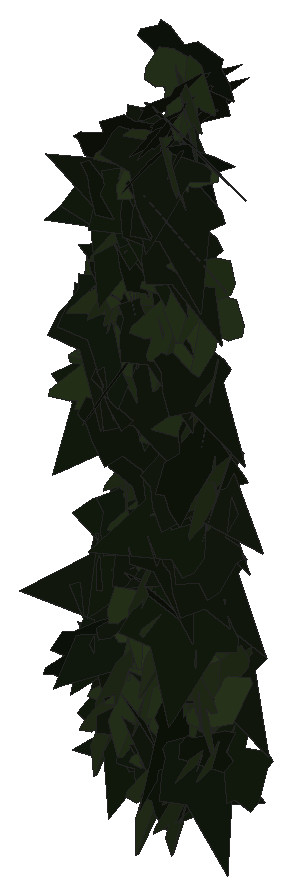
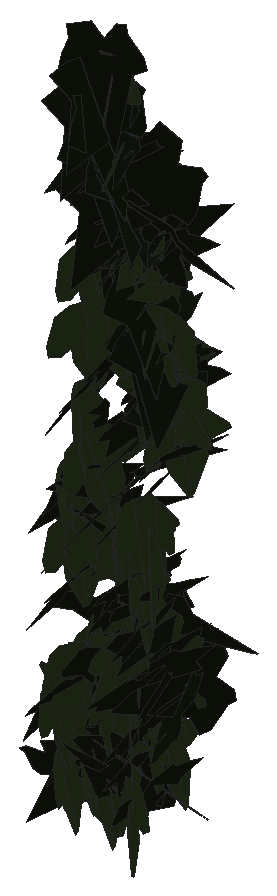
# SketchUp Ruby script. Lengths in inches.
U = 1.inch
M = Sketchup.active_model
def pt(a) = Geom::Point3d.new(a.map { |v| v * U })
def face(e, loops, mat)
  f = e.add_face(loops[0].map { |a| pt(a) })
  loops[1..].each { |l| e.add_face(l.map { |a| pt(a) }).erase! }
  f.material = f.back_material = mat if mat
  f
end
# faces: each face lists its corners as indices into pts; further lists are holes
def faces(e, pts, list, mat = nil) = list.each { |f| face(e, (f[0].is_a?(Array) ? f : [f]).map { |l| l.map { |i| pts[i] } }, mat) }
# xy, xz, yz: faces in a plane at the given z, y or x. An outline is a flat list of corners, or four numbers for a rectangle; further outlines are holes
def ring(l) = l.size == 4 ? [[l[0], l[1]], [l[2], l[1]], [l[2], l[3]], [l[0], l[3]]] : l.each_slice(2).to_a
def flat(e, list, mat, &to3) = list.each { |f| face(e, (f[0].is_a?(Array) ? f : [f]).map { |l| ring(l).map { |u, v| to3.(u, v) } }, mat) }
def xy(e, z, list, mat = nil) = flat(e, list, mat) { |x, y| [x, y, z] }
def xz(e, y, list, mat = nil) = flat(e, list, mat) { |x, z| [x, y, z] }
def yz(e, x, list, mat = nil) = flat(e, list, mat) { |y, z| [x, y, z] }
def lines(e, pts, list) = list.each { |a, b| e.add_line(pt(pts[a]), pt(pts[b])) }
# prism: a flat outline (further loops are holes) pulled along v
def prism(e, loops, v, mat = nil)
  f = face(e, loops, mat); d = Geom::Vector3d.new(v.map { |x| x * U })
  f.pushpull(f.normal.samedirection?(d) ? d.length : -d.length)
end
def box(e, o, s, mat = nil) = prism(e, [[o, [o[0] + s[0], o[1], o[2]], [o[0] + s[0], o[1] + s[1], o[2]], [o[0], o[1] + s[1], o[2]]]], [0, 0, s[2]], mat)
def at(x, y, z, deg = 0) = Geom::Transformation.translation(pt([x, y, z])) * Geom::Transformation.rotation(ORIGIN, Z_AXIS, deg.degrees)
def axes(o, x, y, z) = Geom::Transformation.new([*x, 0, *y, 0, *z, 0, *pt(o).to_a, 1])
def part(name) = M.definitions.add(name)
# library, detail: a bought-in or finely detailed component or shape, given as its bounding box
def library(name, o, s) = part(name).tap { |d| box(d.entities, o, s) }
def detail(e, o, s) = box(e.add_group.entities, o, s)
def put(e, d, t, mat = nil) = e.add_instance(d, t).tap { |i| i.material = mat if mat }
def group(e, t, mat = nil) = e.add_group.tap { |g| g.transformation = t; g.material = mat if mat }.entities
root = M.entities
M.materials.add("efeu1").color = [18, 25, 13]
M.materials.add("efeu2").color = [43, 57, 29]
c1 = part("ivyleaf_9")
p = [[1.54,2.16,1.25],[1.36,2.04,1.19],[-0.21,0.99,0.68],[-0.71,1.11,0.82],[-0.85,0.86,0.67],[-0.8,0.17,0.21],
  [-0.9,-0.01,0.1],[-0.67,-0.16,-0.02],[-0.08,-0.08,-0.05],[-0.03,-0.6,-0.4],[0.65,-0.88,-0.66],[0.83,-0.6,-0.49],
  [1.29,-0.42,-0.43],[1.8125,-0.07,-0.26],[1.21,0.44,0.15]]
faces(c1.entities,p,[[0,1,2,3,4,5,6,7,8,9,10,11,12,13,14]],"efeu1")
c2 = part("ivyleaf_10")
p = [[0,0.5,-0.03],[-0.0625,2.02,-0.43],[-0.19,2.01,-0.46],[-0.54,1.05,-0.29],[-0.52,0.625,-0.18],[-0.83,0.76,-0.28],
  [-1.16,0.64,-0.33],[-1.15,0.33,-0.24],[-0.77,-0.39,0.02],[-0.3,-0.51,0.16],[0.04,-0.48,0.23],[-0.02,2.01,-0.4375],
  [-0.06,2.01,-0.43],[0.04,-0.49,0.23],[0.67,-0.49,0.14],[1.38,0.36,-0.2],[1.375,0.51,-0.24],[0.81,0.65,-0.19],
  [0.62,0.59,-0.15],[0.6,1.09,-0.28],[0.5,1.23,-0.31]]
faces(c2.entities,p,[[0,1,2,3,4,5,6,7,8,9,10],[11,12,0,13,14,15,16,17,18,19,20]],"efeu2")
put(root,c1,axes([14.96,224.05,229.89],[0.063,0.49565,0.01912],[-0.02815,0.02282,-0.49869],[-0.49522,0.06176,0.03078]))
put(root,c1,axes([15.22,223.91,225.72],[-0.39113,0.07566,0.30215],[-0.30173,0.02832,-0.39769],[-0.07729,-0.49343,0.0235]))
put(root,c2,axes([14.84,224.45,226.98],[0.34673,-0.34178,-0.11385],[0.0087,0.16592,-0.47159],[0.36014,0.32505,0.12101]))
put(root,c2,axes([15.23,223.79,228.77],[-0.07541,0.02724,0.49353],[-0.4942,-0.01303,-0.0748],[0.00879,-0.49909,0.02889]))
put(root,c2,axes([14.91,223.86,228.55],[-0.22304,-0.43361,0.11063],[0.0193,-0.13282,-0.48165],[0.44708,-0.21058,0.07599]))
put(root,c1,axes([14.65,223.47,224.73],[0.28736,0.2041,0.35464],[0.2644,0.23812,-0.35128],[-0.31228,0.38942,0.02893]))
put(root,c1,axes([14.9,224.4,225.13],[-0.24918,-0.40137,0.16373],[-0.04775,-0.16229,-0.47051],[0.43085,-0.25012,0.04255]))
put(root,c2,axes([14.92,224.08,223.89],[0.07183,-0.47806,0.12768],[0.03312,-0.12408,-0.48323],[0.4937,0.07788,0.01384]))
put(root,c2,axes([14.95,224.15,227.26],[0.34077,-0.30537,-0.20156],[-0.04793,0.23581,-0.43829],[0.36274,0.31803,0.13144]))
put(root,c1,axes([14.82,224.625,223.45],[-0.09691,-0.47403,0.12613],[-0.01843,-0.12496,-0.48378],[0.49017,-0.09841,0.00674]))
put(root,c1,axes([14.93,224.125,228.18],[-0.28894,-0.35601,0.19943],[-0.00668,-0.2402,-0.43847],[0.408,-0.25605,0.13405]))
put(root,c2,axes([14.75,224.14,229.35],[0.32621,0.31913,0.2043],[0.11757,0.17103,-0.45489],[-0.36022,0.34482,0.03654]))
put(root,c2,axes([14.93,224.78,223.4],[0.37932,-0.2878,-0.1526],[-0.0287,0.20379,-0.45568],[0.32449,0.35446,0.13808]))
put(root,c2,axes([14.99,224.04,229.71],[-0.15997,-0.46885,0.06775],[0.00767,-0.07406,-0.49442],[0.47366,-0.15715,0.03088]))
put(root,c1,axes([14.625,224.17,224.48],[0.31864,-0.36062,0.13572],[0.08272,-0.10799,-0.48114],[0.37633,0.32907,-0.00916]))
put(root,c1,axes([14.86,224.1,229.35],[-0.1462,-0.47355,-0.06618],[0.00774,0.06685,-0.49545],[0.47809,-0.14589,-0.01222]))
put(root,c2,axes([15.01,224.49,226.56],[0.11234,-0.48242,-0.06822],[0.0009,0.07022,-0.49504],[0.48722,0.1111,0.01665]))
put(root,c2,axes([14.98,223.97,229.91],[0.36157,-0.34351,-0.03562],[-0.02197,0.02859,-0.4987],[0.34465,0.3622,0.00558]))
put(root,c1,axes([15.11,224,229.86],[0.03322,0.48974,0.09515],[-0.013,0.09618,-0.49049],[-0.49873,0.03011,0.01912]))
put(root,c1,axes([14.98,224.51,226.22],[-0.25217,-0.40835,0.1402],[0.00224,-0.1636,-0.47247],[0.43174,-0.23766,0.08434]))
put(root,c2,axes([14.91,224.1,230.11],[-0.45836,-0.03724,-0.19626],[0.19586,0.01291,-0.45986],[0.03932,-0.49844,0.00275]))
put(root,c1,axes([15.06,224.125,225.07],[-0.22004,-0.33771,0.29586],[-0.11073,-0.27849,-0.40023],[0.43511,-0.24166,0.04777]))
put(root,c2,axes([15.07,224.04,229.9375],[0.05078,-0.49639,-0.03196],[-0.00004,0.03212,-0.49897],[0.49741,0.05068,0.00322]))
put(root,c2,axes([15.2,224.04,224.49],[-0.39676,-0.25674,0.1633],[-0.12856,-0.10177,-0.47235],[0.27578,-0.41681,0.01474]))
put(root,c1,axes([14.93,224.03,224.83],[0.2535,-0.32237,-0.28603],[-0.19108,0.21337,-0.40983],[0.3863,0.31709,-0.01502]))
put(root,c1,axes([14.92,224.09,229.53],[-0.05922,-0.4947,-0.042],[-0.0005,0.04235,-0.4982],[0.49648,-0.05896,-0.00551]))
put(root,c2,axes([15.03,224.11,229.85],[0.38856,-0.30945,-0.05711],[0.00482,0.09658,-0.49056],[0.31464,0.38067,0.07804]))
put(root,c2,axes([15.13,224.41,227.34],[-0.02667,-0.49752,-0.04199],[-0.01602,0.04288,-0.4979],[0.49903,-0.02521,-0.01822]))
put(root,c2,axes([15.13,224.02,230.03],[-0.28656,0.40933,0.01831],[-0.0453,-0.00944,-0.49785],[-0.40722,-0.28699,0.0425]))
put(root,c1,axes([14.91,224.4,225.87],[0.14941,-0.47135,-0.0742],[-0.01358,0.07352,-0.49438],[0.47696,0.14974,0.00917]))
put(root,c2,axes([15.17,224,225.18],[0.34578,0.35267,0.07784],[-0.05693,-0.0532,0.49389],[0.35664,-0.35042,0.00336]))
put(root,c1,axes([15.48,223.85,231.43],[-0.45026,0.12068,0.18083],[-0.17917,0.02955,-0.46586],[-0.12312,-0.48432,0.01663]))
put(root,c1,axes([15.32,223.98,230.52],[-0.07005,0.49485,0.01483],[-0.00112,0.01482,-0.49978],[-0.49507,-0.07005,-0.00097]))
put(root,c1,axes([14.96,224.4,223.91],[0.12104,-0.47489,-0.09916],[-0.00343,0.10136,-0.48961],[0.48512,0.1192,0.02128]))
put(root,c2,axes([15.22,224.37,224.14],[0.18163,-0.42331,-0.19447],[-0.02706,0.19879,-0.45799],[0.46506,0.1769,0.0493]))
put(root,c1,axes([14.86,224,230.07],[0.31194,-0.38416,0.07154],[0.08818,-0.01997,-0.49176],[0.38068,0.31941,0.05529]))
put(root,c1,axes([15.01,224.37,224.29],[0.05807,-0.49533,-0.03577],[-0.00035,0.03597,-0.4987],[0.49662,0.05794,0.00383]))
put(root,c1,axes([15.5625,224.29,223.56],[-0.40912,0.21874,0.18648],[-0.21023,-0.00648,-0.45361],[-0.19603,-0.44957,0.09727]))
put(root,c1,axes([15.52,223.99,231.15],[-0.04477,-0.00173,0.49799],[-0.49581,-0.04663,-0.04474],[0.0466,-0.49782,0.00246]))
put(root,c1,axes([15.23,223.39,228.59],[0.16105,0.15924,0.44576],[0.07656,0.45589,-0.19052],[-0.46712,0.12962,0.12246]))
put(root,c1,axes([15,224.58,225.02],[0.15008,-0.43164,-0.2029],[0.05278,0.22643,-0.44266],[0.47402,0.11145,0.11353]))
put(root,c1,axes([15.23,224,231.19],[-0.2588,-0.42569,-0.04263],[0.01166,0.04278,-0.49803],[0.42765,-0.25877,-0.01221]))
put(root,c2,axes([15.3,223.84,224.73],[0.05533,-0.48125,-0.12383],[0.00234,0.12485,-0.48416],[0.49692,0.05299,0.01607]))
put(root,c1,axes([15.03,224.4,226.55],[0.13227,-0.45362,-0.16352],[0.05024,0.1816,-0.46314],[0.47956,0.10608,0.09362]))
put(root,c1,axes([15.04,223.73,228.23],[0.33176,-0.32221,-0.19004],[-0.04944,0.21401,-0.44917],[0.37079,0.31683,0.11014]))
put(root,c1,axes([15.02,223.86,231.39],[0.27702,-0.41617,-0.00811],[0.02374,0.02552,-0.49878],[0.41557,0.27596,0.0339]))
put(root,c1,axes([15.08,223.9375,228.7],[0.34175,-0.29492,-0.215],[-0.06128,0.244,-0.4321],[0.35979,0.32169,0.13063]))
put(root,c2,axes([15.42,224.03,224.29],[-0.23049,-0.40968,0.17039],[-0.04048,-0.17179,-0.46781],[0.44185,-0.22945,0.04603]))
put(root,c2,axes([15.25,223.87,230.37],[0.06203,0.46464,0.17395],[0.00299,0.17496,-0.46838],[-0.49613,0.05915,0.01892]))
put(root,c2,axes([15.38,223.95,230.77],[-0.12653,-0.48363,-0.00932],[0.00861,0.00739,-0.49987],[0.48365,-0.12666,0.00646]))
put(root,c2,axes([15.68,223.76,229.91],[-0.19398,0.08933,0.45209],[-0.44008,0.10966,-0.2105],[-0.13676,-0.47958,0.03608]))
put(root,c2,axes([15.41,223.74,231.4375],[-0.42031,0.26851,0.03522],[-0.02788,0.02178,-0.49875],[-0.26937,-0.42122,-0.00334]))
put(root,c1,axes([15.2,223.55,232.23],[0.42415,0.24786,0.09305],[0.07591,0.05451,-0.49119],[-0.25364,0.43081,0.00861]))
put(root,c1,axes([15.27,223.89,225.75],[0.48899,0.03144,-0.09949],[-0.10025,0.00931,-0.48976],[-0.02894,0.49892,0.0154]))
put(root,c2,axes([15.5,224.4375,227.15],[0.24738,-0.41812,-0.11822],[-0.00802,0.13161,-0.4823],[0.43444,0.24052,0.05841]))
put(root,c1,axes([15.31,224.32,226.12],[0.10396,-0.47974,-0.09512],[-0.02018,0.09295,-0.49087],[0.48866,0.1059,-0.00004]))
put(root,c2,axes([15.44,224.45,224.76],[-0.0517,-0.497,-0.01789],[0.13194,0.00364,-0.48226],[0.4795,-0.05458,0.13077]))
put(root,c1,axes([15.74,223.88,231.65],[-0.06364,0.32749,0.37243],[-0.12111,0.35385,-0.33185],[-0.48092,-0.13245,0.03429]))
put(root,c2,axes([15.44,224.24,225.17],[-0.13231,-0.41582,-0.24411],[0.1646,0.19897,-0.42816],[0.45321,-0.19366,0.08423]))
put(root,c2,axes([15.57,224.13,226.82],[-0.14471,-0.4665,0.10696],[0.0135,-0.11567,-0.48625],[0.47841,-0.13785,0.04608]))
put(root,c2,axes([15.46,223.92,225.77],[0.16078,0.46854,-0.06796],[-0.02279,-0.06403,-0.49536],[-0.47289,0.16239,0.00076]))
put(root,c1,axes([15.34,224.31,227.35],[0.04849,-0.47885,0.13546],[0.03554,-0.13242,-0.48084],[0.49637,0.05626,0.0212]))
put(root,c1,axes([15.35,223.97,228.71],[0.12415,-0.42572,-0.23098],[-0.02098,0.23349,-0.44163],[0.48389,0.11935,0.04011]))
put(root,c1,axes([15.29,224.07,230.38],[0.29404,-0.40268,-0.0373],[0.0021,0.04764,-0.49772],[0.4044,0.29254,0.0297]))
put(root,c2,axes([15.66,223.84,232.14],[-0.24462,-0.42699,0.08857],[-0.04146,-0.07832,-0.49208],[0.4341,-0.24809,0.00291]))
put(root,c2,axes([15.5625,223.93,231.15],[0.30748,-0.37279,-0.12837],[0.01313,0.17238,-0.46916],[0.39406,0.28515,0.1158]))
put(root,c1,axes([15.31,224.4,223.72],[-0.08746,-0.21798,-0.4414],[0.29209,0.3379,-0.22474],[0.39628,-0.29716,0.06823]))
put(root,c2,axes([15.625,223.94,226.15],[0.13585,-0.46529,-0.12267],[-0.0067,0.12562,-0.48392],[0.48114,0.13313,0.02789]))
put(root,c1,axes([15.51,224.5625,225.32],[-0.15778,-0.4632,-0.1027],[0.02669,0.09939,-0.48929],[0.4737,-0.15989,-0.00664]))
put(root,c2,axes([15.76,224.32,224.04],[-0.36318,-0.31795,0.13042],[-0.06481,-0.12297,-0.48029],[0.33749,-0.36577,0.04811]))
put(root,c1,axes([15.5,223.95,231.13],[-0.20832,-0.26151,-0.37177],[0.21863,0.3009,-0.33416],[0.3985,-0.30178,-0.01102]))
put(root,c1,axes([15.9,223.8,232.17],[-0.14646,0.47759,-0.02148],[-0.00766,-0.02481,-0.49933],[-0.47801,-0.14593,0.01458]))
put(root,c2,axes([15.87,224.33,223.29],[-0.34047,-0.32694,0.16489],[-0.06008,-0.17222,-0.46554],[0.36121,-0.33682,0.07799]))
put(root,c2,axes([15.78,224.19,225.24],[0.06453,-0.41082,0.27761],[0.03277,-0.2758,-0.41576],[0.49473,0.07185,-0.00867]))
put(root,c1,axes([15.7,223.96,231.86],[0.38977,0.31209,-0.02616],[-0.02324,-0.01283,-0.49929],[-0.31232,0.39043,0.0045]))
put(root,c1,axes([15.62,223.85,231.48],[-0.13947,-0.42677,-0.22003],[0.12088,0.19053,-0.44619],[0.46469,-0.17765,0.05003]))
put(root,c2,axes([15.77,223.9,223.21],[0.06768,-0.45034,0.20644],[0.07349,-0.19692,-0.45368],[0.48992,0.09175,0.03953]))
put(root,c1,axes([15.54,223.95,231.14],[0.2124,-0.45202,0.02381],[0.02762,-0.01331,-0.49906],[0.4518,0.21331,0.01931]))
put(root,c1,axes([15.59,223.85,231.38],[0.3648,-0.33703,-0.05769],[-0.0359,0.04614,-0.49657],[0.34004,0.36644,0.00947]))
put(root,c2,axes([15.79,223.86,231.87],[0.3347,0.37125,0.01226],[-0.03446,0.04747,-0.49655],[-0.36985,0.33155,0.05736]))
put(root,c2,axes([15.94,224.34,228.05],[-0.17839,-0.45179,0.11858],[-0.02946,-0.1158,-0.48551],[0.46617,-0.18021,0.0147]))
put(root,c1,axes([15.65,223.96,229.6],[0.13909,-0.46775,-0.10892],[-0.00582,0.11174,-0.48732],[0.48023,0.13683,0.02564]))
put(root,c1,axes([16.01,223.85,232.52],[0.03431,0.49876,-0.00806],[-0.03105,-0.00592,-0.499],[-0.49785,0.03474,0.03057]))
put(root,c1,axes([15.79,223.95,232.21],[-0.1398,-0.47977,-0.01663],[-0.00039,0.01743,-0.4997],[0.48006,-0.1397,-0.00525]))
put(root,c2,axes([15.95,223.8,232.22],[-0.25662,0.41554,0.10711],[-0.05842,0.08981,-0.48839],[-0.42513,-0.26318,0.00246]))
put(root,c1,axes([16.11,224.08,226.9],[-0.32128,-0.17266,0.342],[-0.21615,-0.28682,-0.34787],[0.31631,-0.37138,0.10966]))
put(root,c1,axes([15.6,223.85,231.26],[0.42068,-0.24067,0.1229],[0.10792,-0.05885,-0.48466],[0.24775,0.4343,0.00243]))
put(root,c1,axes([15.72,223.96,226.64],[0.17829,-0.46656,-0.02303],[-0.00476,0.02284,-0.49946],[0.46711,0.17832,0.0037]))
put(root,c2,axes([16.03,224.3,226.85],[-0.09062,-0.42558,0.24632],[-0.03524,-0.2442,-0.43488],[0.49046,-0.09618,0.01427]))
put(root,c1,axes([16.14,223.79,232.74],[-0.1165,0.48623,-0.00331],[0.00724,-0.00167,-0.49994],[-0.48618,-0.11654,-0.00665]))
put(root,c2,axes([15.98,223.95,229.79],[-0.06386,-0.46204,0.18012],[0.04968,-0.18665,-0.46119],[0.49341,-0.04101,0.06974]))
put(root,c1,axes([15.91,224.11,224.25],[-0.12388,0.13102,-0.46635],[0.33293,-0.32662,-0.1802],[-0.35187,-0.35518,-0.00631]))
put(root,c1,axes([15.75,224.41,227.24],[0.27197,-0.38452,-0.16786],[-0.02704,0.18356,-0.4643],[0.41869,0.26163,0.07905]))
put(root,c2,axes([16.03,224.04,223.04],[0.11478,-0.48576,-0.02942],[-0.00745,0.02847,-0.49913],[0.48659,0.11502,-0.00071]))
put(root,c2,axes([16,224.35,224.44],[-0.15751,-0.40575,-0.24609],[0.11962,0.21697,-0.4343],[0.45922,-0.19568,0.02872]))
put(root,c2,axes([16.08,224.16,223.375],[0.12782,-0.48317,0.01451],[-0.00171,-0.01546,-0.49976],[0.48338,0.1277,-0.0056]))
put(root,c2,axes([16.15,224.43,226.8],[-0.18467,-0.46257,0.04393],[-0.00927,-0.0436,-0.49801],[0.46456,-0.18474,0.00753]))
put(root,c2,axes([16.18,224.29,224.18],[0.4583,0.05225,0.19295],[-0.19134,-0.02504,0.46126],[0.05787,-0.49663,-0.00295]))
put(root,c2,axes([16.19,224.71,224.46],[-0.01086,-0.49988,0.00225],[-0.00054,-0.00223,-0.49999],[0.49988,-0.01086,-0.00049]))
put(root,c2,axes([16.21,224.15,229.83],[-0.33614,-0.35609,0.10104],[0.01168,-0.14663,-0.47787],[0.36997,-0.3189,0.10689]))
put(root,c1,axes([15.87,223.78,232.59],[0.47944,-0.14102,0.01573],[0.02463,0.02812,-0.4986],[0.13975,0.47888,0.03391]))
put(root,c1,axes([16.28,223.69,233.78],[0.29927,0.16321,-0.36579],[-0.32193,-0.17368,-0.34088],[-0.23833,0.43954,0.00113]))
put(root,c2,axes([16.16,224.64,223.42],[0.13328,-0.48109,0.02806],[0.03482,-0.01942,-0.49841],[0.48065,0.13481,0.02832]))
put(root,c1,axes([16.2,223.59,233.12],[0.21047,0.42538,0.15733],[-0.00157,0.17413,-0.4687],[-0.45354,0.1968,0.07464]))
put(root,c2,axes([16.21,224.25,228.65],[0.14551,-0.46527,-0.11115],[-0.01574,0.11146,-0.48716],[0.4781,0.14527,0.01779]))
put(root,c1,axes([16.21,223.76,232.83],[0.18366,0.4372,0.15851],[0.0133,0.16541,-0.47166],[-0.46486,0.17746,0.04912]))
put(root,c1,axes([16.08,223.91,223.45],[-0.01098,-0.03363,-0.49875],[-0.08876,0.49107,-0.03116],[0.49194,0.08785,-0.01675]))
put(root,c1,axes([16.41,224.65,223.47],[-0.48175,-0.12854,0.03739],[-0.03539,-0.0124,-0.49859],[0.1291,-0.48304,0.00285]))
put(root,c1,axes([16.13,224,225.62],[-0.29627,-0.37569,-0.14519],[0.16596,0.05036,-0.46896],[0.36699,-0.32606,0.09486]))
put(root,c1,axes([16,224.69,224.73],[0.16804,-0.43015,-0.19166],[-0.00306,0.20249,-0.45715],[0.47091,0.15481,0.06542]))
put(root,c1,axes([16.52,224.11,226.75],[-0.48223,0.05093,0.12192],[-0.12309,-0.00547,-0.48458],[-0.04802,-0.49737,0.01782]))
put(root,c1,axes([16.02,223.85,231.49],[0.0796,-0.48529,-0.09034],[0.01088,0.09321,-0.49112],[0.4935,0.07622,0.0254]))
put(root,c2,axes([16.25,223.72,233.1875],[-0.36759,0.3384,0.01912],[-0.03835,-0.01349,-0.49834],[-0.33676,-0.36784,0.03587]))
put(root,c2,axes([16.04,224.26,224.97],[0.28384,-0.33066,0.24514],[0.24719,-0.10117,-0.42268],[0.32914,0.36114,0.10604]))
put(root,c2,axes([16.18,223.92,224.76],[-0.40452,0.27538,-0.10261],[0.08225,-0.06151,-0.48934],[-0.28213,-0.41278,0.00447]))
put(root,c1,axes([15.98,224.125,227.6],[0.15015,-0.34544,-0.32882],[0.0562,0.35515,-0.34743],[0.4736,0.06737,0.14548]))
put(root,c1,axes([16.02,223.85,230.95],[0.18454,-0.44189,-0.1438],[-0.01171,0.15025,-0.47675],[0.46455,0.17932,0.0451]))
put(root,c2,axes([16.33,224.3,224.71],[-0.10235,-0.4853,-0.06327],[-0.00018,0.06468,-0.4958],[0.48941,-0.10147,-0.01341]))
put(root,c1,axes([16.05,224.06,229.08],[0.25243,-0.39745,-0.16827],[-0.03994,0.17258,-0.46757],[0.42975,0.2495,0.05538]))
put(root,c1,axes([16.28,223.67,228.03],[0.10212,-0.04166,-0.48768],[-0.26929,0.41123,-0.09152],[0.40872,0.28135,0.06155]))
put(root,c2,axes([16.25,223.6875,233.42],[0.49158,-0.08598,-0.03095],[-0.0084,0.12613,-0.48376],[0.09099,0.47613,0.12256]))
put(root,c2,axes([16.32,224.37,227.49],[0.13495,-0.48027,0.03359],[0.00452,-0.03362,-0.49885],[0.48142,0.13494,-0.00473]))
put(root,c1,axes([16.06,224.27,226.22],[0.24232,-0.38357,-0.21014],[-0.01397,0.23333,-0.442],[0.43714,0.22008,0.10236]))
put(root,c2,axes([16.39,223.84,230.55],[-0.24267,-0.42094,0.11797],[-0.02539,-0.12113,-0.48444],[0.43643,-0.24111,0.03742]))
put(root,c1,axes([16.15,224.17,223.46],[0.11868,-0.47448,-0.10386],[-0.02935,0.09971,-0.48908],[0.48482,0.12218,-0.00419]))
put(root,c2,axes([16.34,224.14,227.44],[0.12118,-0.43395,-0.2168],[0.03816,0.2313,-0.44164],[0.48359,0.09049,0.08918]))
